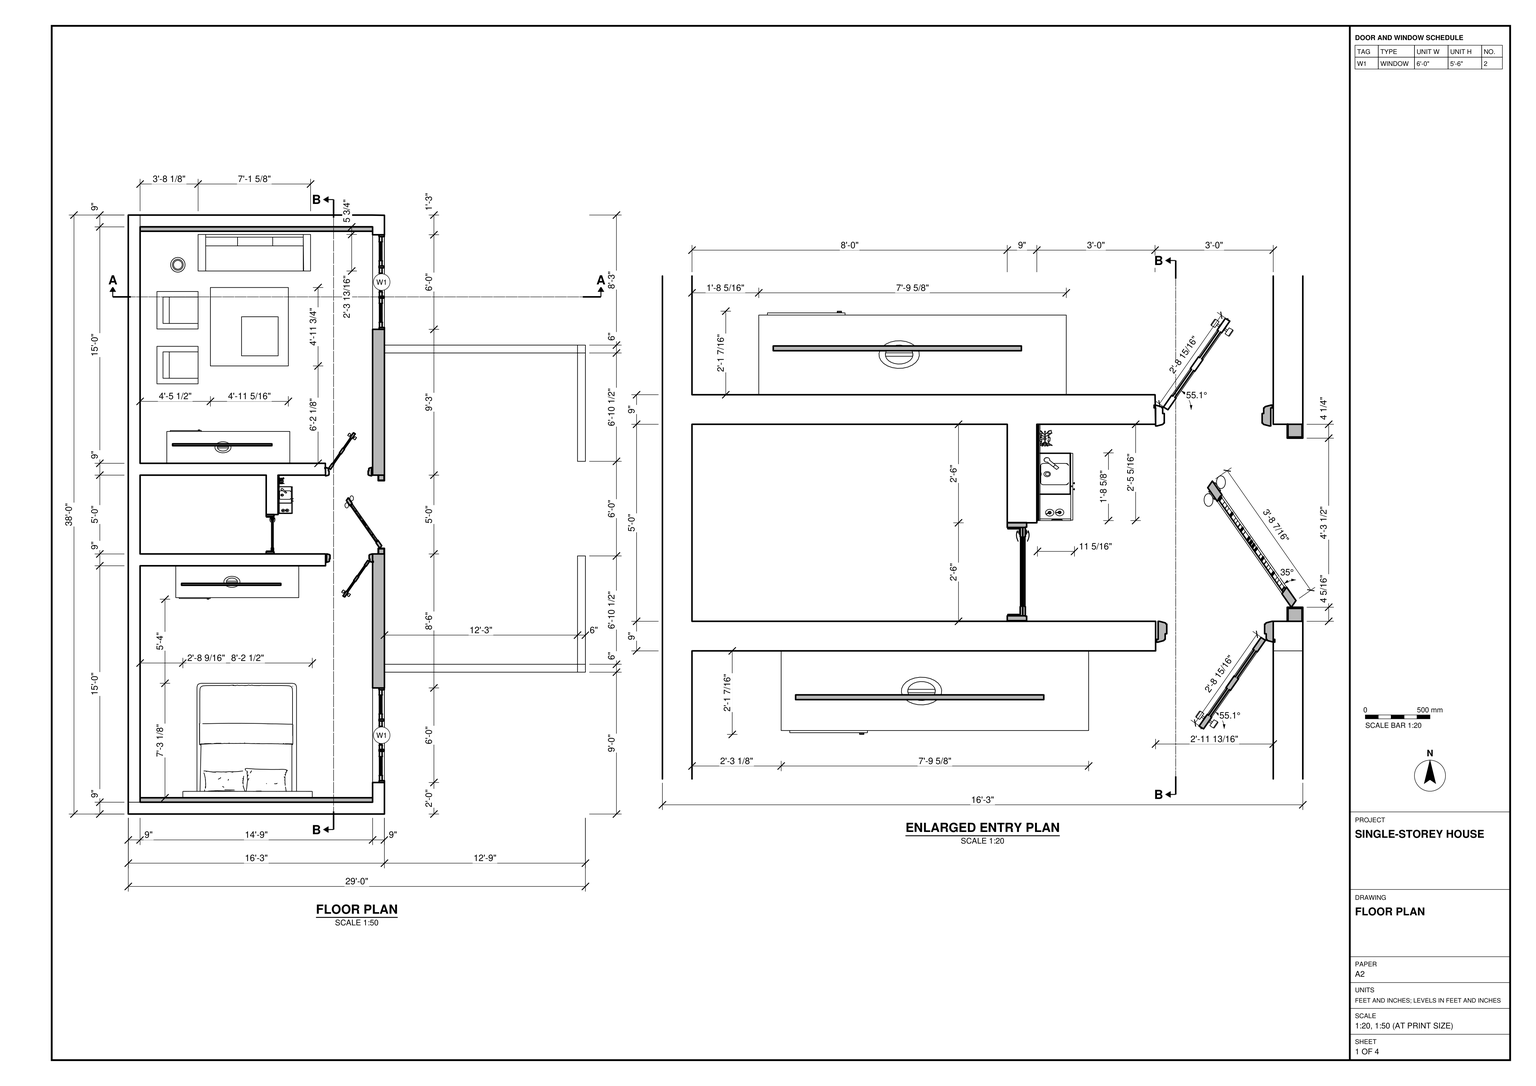
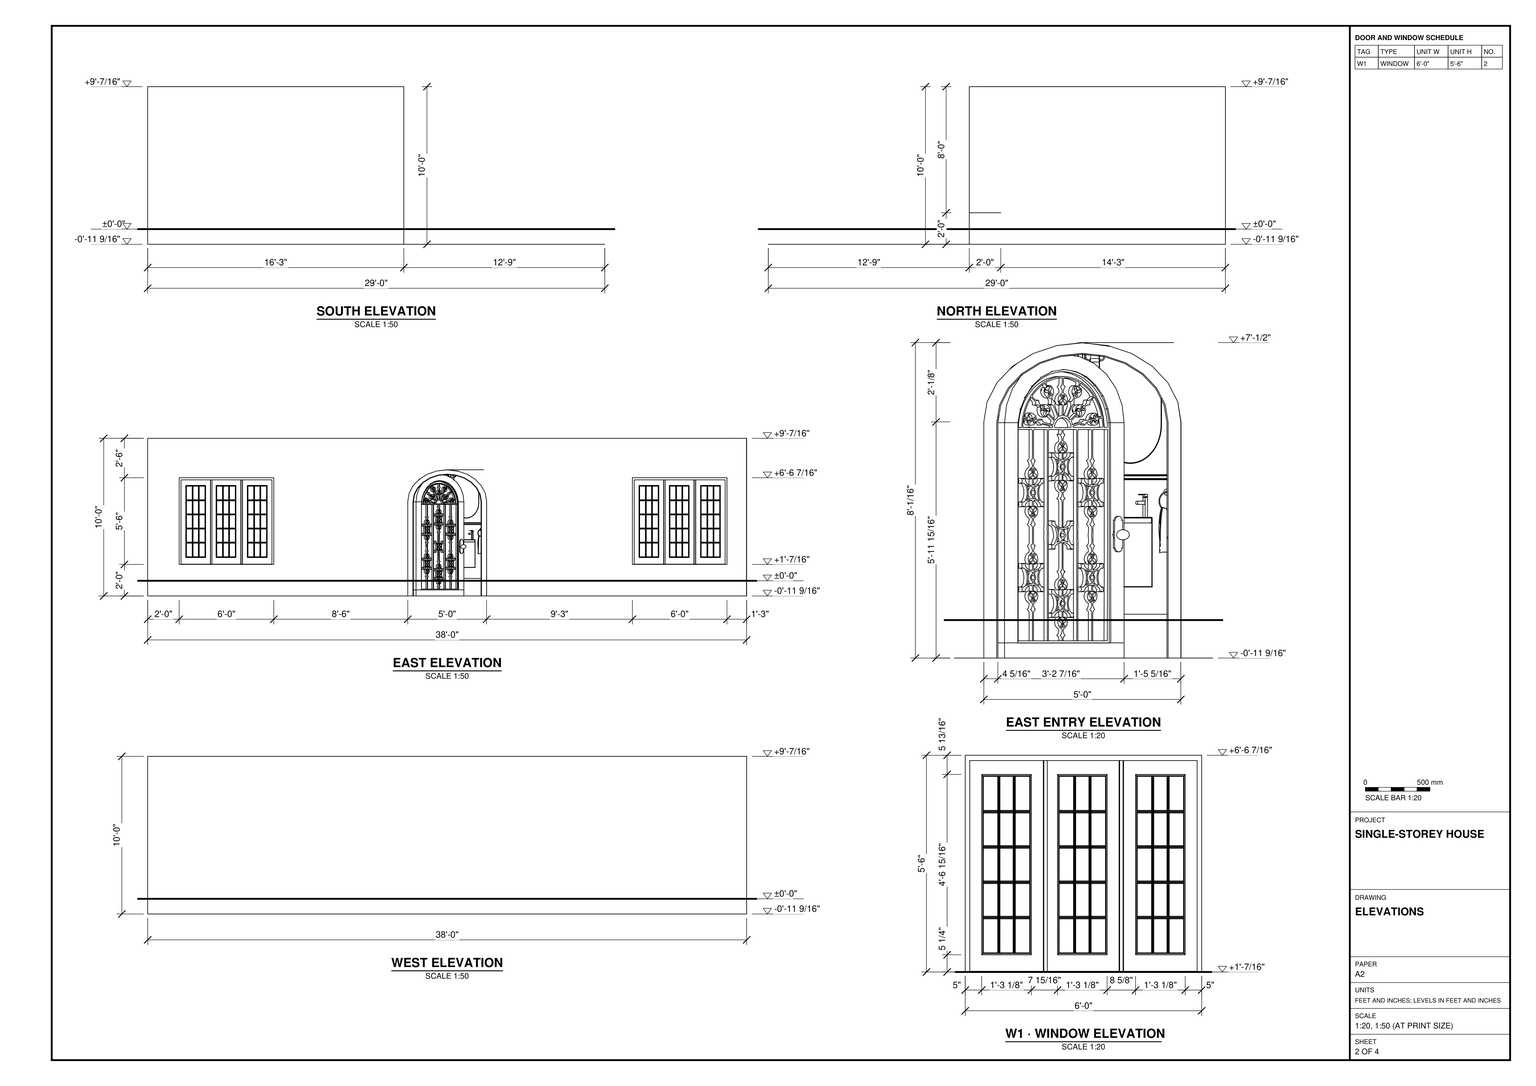
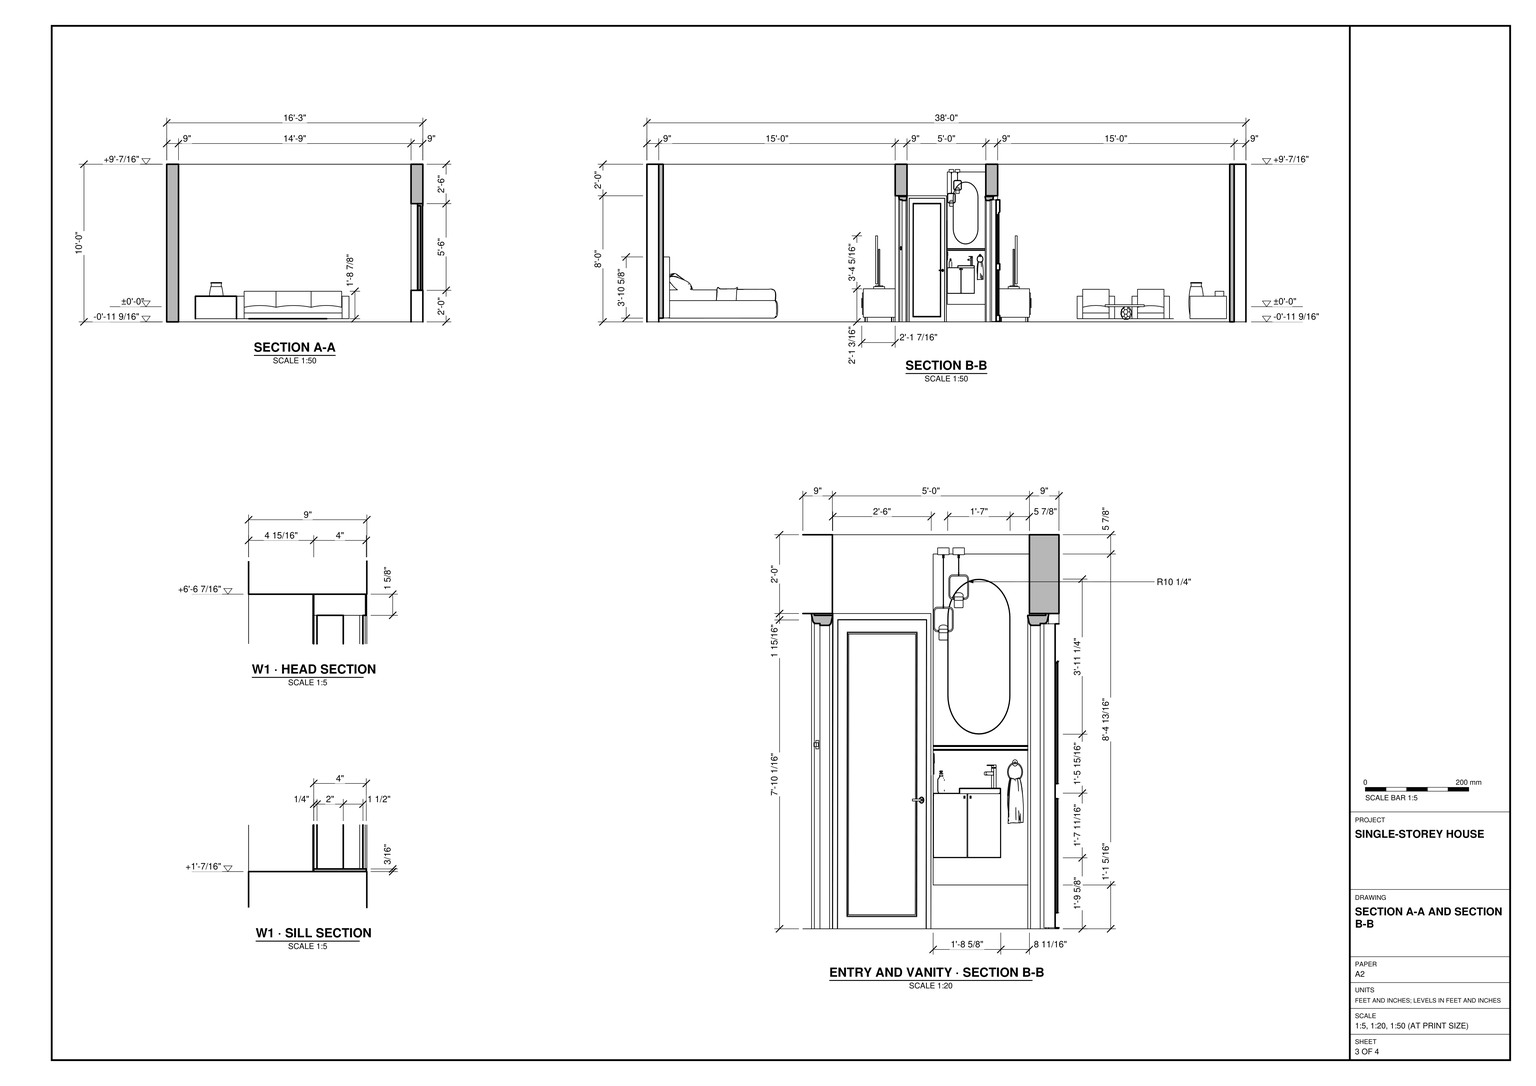
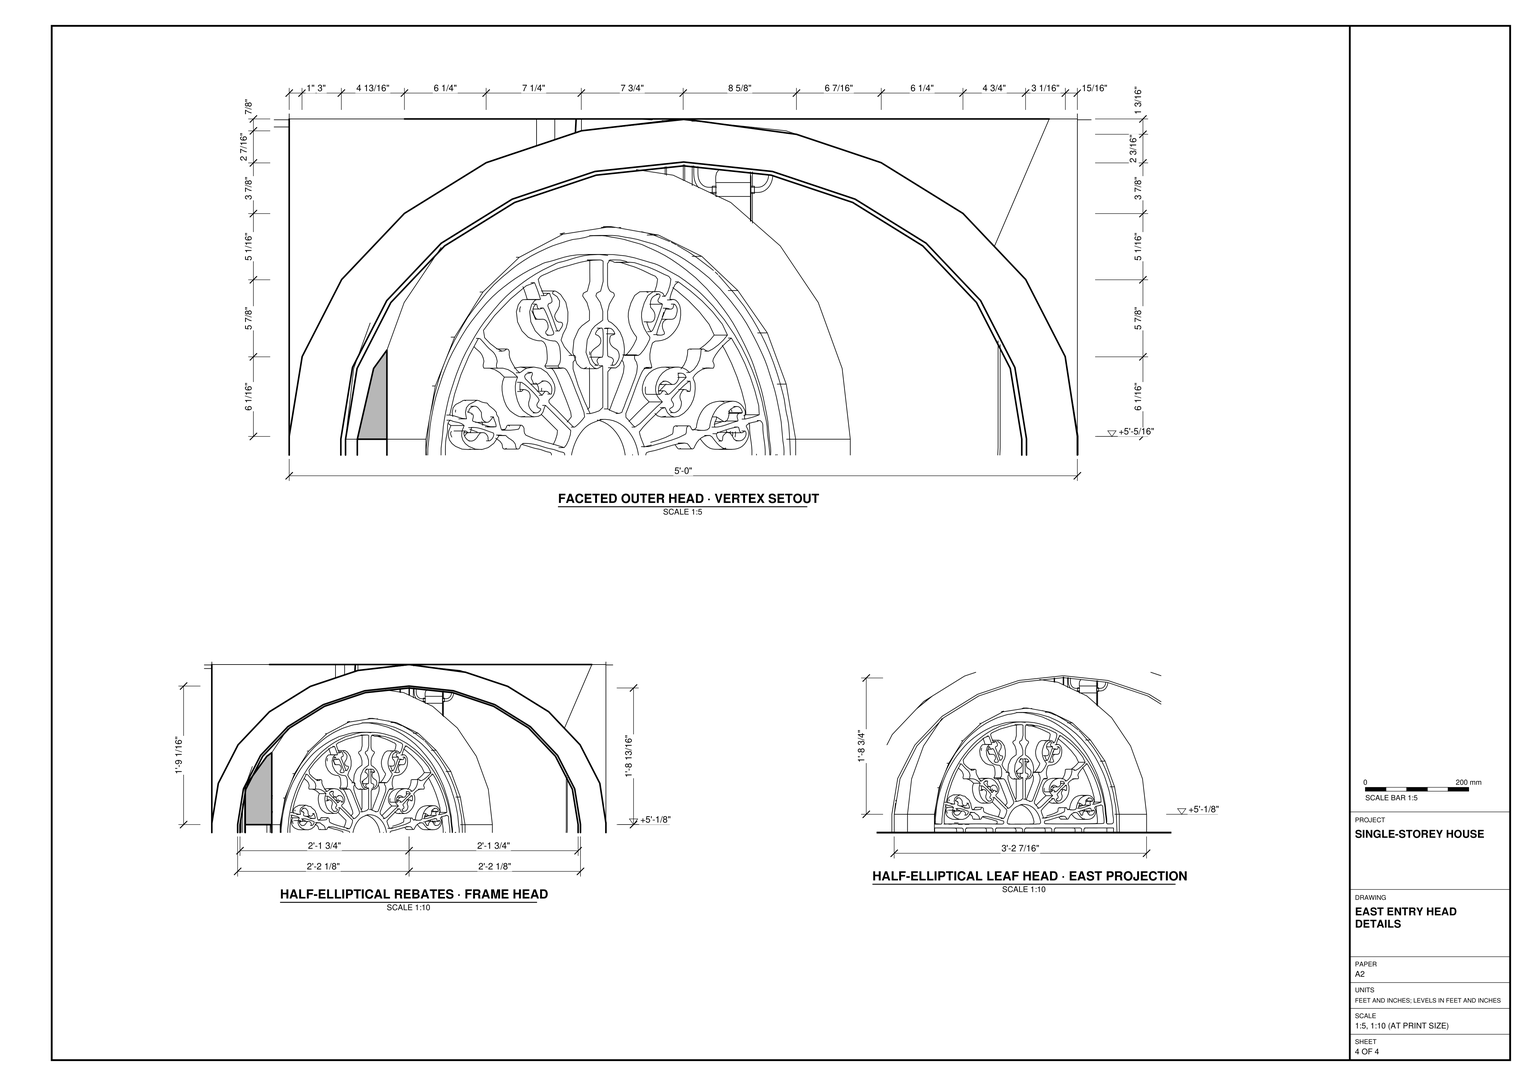
Build the house shown in task_files/diagram_01.pdf in SketchUp. Work in feet and inches. Use ±0'-0" as the ground-floor datum and follow the sections for the wall tops, window sills and floor position relative to that datum. The overall model is 29'-0" wide, 38'-0" long and 10'-0" high. The enclosed house is 16'-3" wide; the outline projecting from its east side accounts for the rest of the width. Follow the plan for its returns and the gap opposite the entrance.

Model the floor and the walls at their drawn thicknesses. Place the living room at the north end and the bedroom at the south end, with the entry and washbasin area between them. Use the enlarged entry plan for the partition returns, door positions and swing directions. Form the arched entrance and place a framed, divided-light window on either side of it, following the east elevation.

Set the sofa against the north wall and arrange the chairs and low table as drawn. Place the bed with its head against the south wall. Fit a television console against each room's entry-side partition, and include the vanity, basin and mirror in the entry recess. Decor and loose items may be any suitable library components. Keep shell elements and individual furniture or joinery pieces in separate groups or components, and use components for repeated parts. Save one SketchUp model as output_files/furnished_single_storey_house_with_arched_entry.skp.

# SketchUp Ruby script. Lengths in inches.
U = 1.inch
M = Sketchup.active_model
def pt(a) = Geom::Point3d.new(a.map { |v| v * U })
def face(e, loops, mat)
  f = e.add_face(loops[0].map { |a| pt(a) })
  loops[1..].each { |l| e.add_face(l.map { |a| pt(a) }).erase! }
  f.material = f.back_material = mat if mat
  f
end
# faces: each face lists its corners as indices into pts; further lists are holes
def faces(e, pts, list, mat = nil) = list.each { |f| face(e, (f[0].is_a?(Array) ? f : [f]).map { |l| l.map { |i| pts[i] } }, mat) }
# xy, xz, yz: faces in a plane at the given z, y or x. An outline is a flat list of corners, or four numbers for a rectangle; further outlines are holes
def ring(l) = l.size == 4 ? [[l[0], l[1]], [l[2], l[1]], [l[2], l[3]], [l[0], l[3]]] : l.each_slice(2).to_a
def flat(e, list, mat, &to3) = list.each { |f| face(e, (f[0].is_a?(Array) ? f : [f]).map { |l| ring(l).map { |u, v| to3.(u, v) } }, mat) }
def xy(e, z, list, mat = nil) = flat(e, list, mat) { |x, y| [x, y, z] }
def xz(e, y, list, mat = nil) = flat(e, list, mat) { |x, z| [x, y, z] }
def yz(e, x, list, mat = nil) = flat(e, list, mat) { |y, z| [x, y, z] }
def lines(e, pts, list) = list.each { |a, b| e.add_line(pt(pts[a]), pt(pts[b])) }
# prism: a flat outline (further loops are holes) pulled along v
def prism(e, loops, v, mat = nil)
  f = face(e, loops, mat); d = Geom::Vector3d.new(v.map { |x| x * U })
  f.pushpull(f.normal.samedirection?(d) ? d.length : -d.length)
end
def box(e, o, s, mat = nil) = prism(e, [[o, [o[0] + s[0], o[1], o[2]], [o[0] + s[0], o[1] + s[1], o[2]], [o[0], o[1] + s[1], o[2]]]], [0, 0, s[2]], mat)
def at(x, y, z, deg = 0) = Geom::Transformation.translation(pt([x, y, z])) * Geom::Transformation.rotation(ORIGIN, Z_AXIS, deg.degrees)
def axes(o, x, y, z) = Geom::Transformation.new([*x, 0, *y, 0, *z, 0, *pt(o).to_a, 1])
def part(name) = M.definitions.add(name)
# library, detail: a bought-in or finely detailed component or shape, given as its bounding box
def library(name, o, s) = part(name).tap { |d| box(d.entities, o, s) }
def detail(e, o, s) = box(e.add_group.entities, o, s)
def put(e, d, t, mat = nil) = e.add_instance(d, t).tap { |i| i.material = mat if mat }
def group(e, t, mat = nil) = e.add_group.tap { |g| g.transformation = t; g.material = mat if mat }.entities
root = M.entities
M.materials.add("[Beadboard]").color = [218, 143, 90]
M.materials.add("[Color M02]").color = [198, 198, 198]
M.materials.add("[Color M05]").color = [114, 114, 114]
M.materials.add("[Color M06]").color = [86, 86, 86]
M.materials.add("[Color_003]8").color = [199, 191, 184]
M.materials.add("[Color_A01]5").color = [191, 191, 191]
M.materials.add("[Color_A01]7").color = [193, 189, 163]
M.materials.add("[Color_A07]3").color = [188, 183, 174]
M.materials.add("[Ornate Tile 01]").color = [202, 202, 202]
c1 = library("BED 7",[-211.22,-92.85,196.6875],[87.15,98.53,46.62])
c2 = library("rack com tv",[110.42,162.32,-6.69],[191.73,75.99,125.98])
c3 = library("sofa set1",[-89.36,-29.2,-0.92],[221.25,236.08,46.83])
c4 = library("Раковина зеркало",[0,0,0],[11.3,36.42,102.67])
c5 = library("Three-panel window",[0.125,0,0],[4,104,82])
c6 = library("Group\#22",[0,0,0],[5.99,4.27,3.3])
c7 = library("Group\#8",[0,0,0],[6.69,30,96])
c8 = library("Group\#6",[-3,-0.25,0],[42,4.75,83.03])
c9 = library("Group\#7",[0,-2.02,0],[36,8.06,80])
xy(root,0,[[195,108,342,114],[342,108,348,114],[342,114,348,196.5],[342,268.5,348,351],[195,351,342,357],
  [342,351,348,357],[186,443.61,186.12,447],[9,443.67,186,447],[9,447,186,447.0625]])
xy(root,0,[[0,9,0,456,9,456,9,267,150,267,150.17,258,114,258,114,228,105,228,105,258,9,258,9,198,150.17,198,150.17,189,9,189,9,9],[186,189,195,198]],"[Color M02]")
xy(root,0,[[150.47,191.65,150.875,191.65,152.53,192.09,152.58,192.11,152.625,192.13,152.67,192.16,152.71,192.19,152.75,192.23,152.78,192.27,152.8125,192.31,152.84,192.36,152.86,192.4,152.875,192.45,152.89,192.51,153.09,192.51,153.09,194.21,153.57,194.21,153.57,197.15,153.36,197.15,153.35,197.2,153.31,197.3,153.28,197.34,153.25,197.39,153.18,197.46,153.1,197.52,153.05,197.54,153,197.5625,151.34,198,150.94,198,150.94,192.51,150.47,192.51],[186.07,191.65,186.47,191.65,186.47,192.51,186,192.51,186,198,185.6,198,183.9375,197.5625,183.89,197.54,183.84,197.52,183.76,197.46,183.69,197.39,183.66,197.34,183.63,197.3,183.61,197.25,183.6,197.2,183.58,197.15,183.37,197.15,183.37,194.21,183.85,194.21,183.85,192.51,184.05,192.51,184.07,192.45,184.08,192.4,184.11,192.36,184.13,192.31,184.16,192.27,184.2,192.23,184.23,192.19,184.27,192.16,184.32,192.13,184.36,192.11,184.41,192.09]],"[Color M05]")
xy(root,2.82,[[9,9,186,12.39]])
xy(root,24,[[186,369,195,441]])
xy(root,24,[[186,24,195,96]],"[Color M02]")
xy(root,54.78,[[153.05,192.97,153.09,193.86]],"[Color M05]")
xy(root,55.49,[[153.05,192.37,153.09,192.51],[153.05,192.51,153.09,192.97],[152.64,193.1,153.05,193.74],[153.05,193.1,153.09,193.74]],"[Color M05]")
xy(root,56.65,[[153.05,192.37,153.09,192.51],[153.05,192.51,153.09,192.97],[152.64,193.1,153.05,193.74],[153.05,193.1,153.09,193.74]],"[Color M05]")
xy(root,57.36,[[153.05,192.97,153.09,193.86]],"[Color M05]")
xy(root,90,[[186,24,195,96],[186,369,195,441]],"[Color M02]")
xy(root,92.4,[[153.57,194.21,183.37,197.15]],"[Color M05]")
xy(root,92.96,[[153.09,192.51,183.85,194.21]],"[Color M05]")
xy(root,95.45,[[150.94,192.51,186,198]],"[Color M05]")
xy(root,96,[[150.17,189,186,198],[105,198,114,228],[150.17,258,150,267,186,267,186,258]])
xy(root,96,[[150.47,191.65,186.47,192.51]],"[Color M05]")
xy(root,96.0625,[[186,198,190,202.32],[186,202.32,190.0625,206.77],[186,206.77,186,258,190.375,258,190.375,255.86,190.5,255.86,190.5,228,190.3125,228,190.3125,219.84,190.25,219.84,190.25,216.83,190.0625,216.83,190.0625,206.77],[190.0625,206.77,195,207.76],[190.0625,207.76,195,210.38],
  [190.0625,210.38,195,215.44],[190.0625,215.44,195,216.83],[190.25,216.83,195,218.22],[190.25,218.22,195,218.41],[190.25,218.41,195,219.84],
  [190.3125,219.84,195,220.25],[190.3125,220.25,195,221.34],[190.3125,221.34,195,228],[190.5,228,194.75,255.86],[190.375,255.86,190.5,258],
  [190.5,255.86,190.8125,258]])
xy(root,120,[[9,9,186,12.39],[9,447,186,447.0625]])
xy(root,120,[[[0,0,186,0,186,9,9,9,9,189,186,189,186,114,195,114,195,258,186,258,186,198,114,198,114,258,195,258,195,351,186,351,186,267,9,267,9,447.0625,186,447.0625,186,357,195,357,195,455.85,186,456,0,456],[9,198,105,258]],[186,0,195,108],[186,108,195,114],[186,351,195,357]],"[Color M02]")
xy(root,120.01,[[9,443.67,186,447.0625]])
xz(root,0,[[0,0,186,120],[186,0,195,120]])
xz(root,9,[[9,0,186,2.82]])
xz(root,9,[[9,2.82,186,120]],"[Color_A01]7")
xz(root,12.39,[[9,2.82,186,120]],"[Color_A01]5")
xz(root,24,[[186,24,195,90]],"[Color M02]")
xz(root,96,[[186,24,195,90]],"[Color M02]")
xz(root,189,[[9,0,150.17,0,150.17,96,186,96,186,120,9,120]],"[Color M02]")
xz(root,191.65,[[150.47,0,150.47,96,186.47,96,186.47,0,186.07,0,186.07,95.53,150.875,95.53,150.875,0]],"[Color M05]")
xz(root,192.37,[[153.05,55.49,153.09,56.65]],"[Color M05]")
xz(root,192.51,[[150.47,0,150.94,0,150.94,95.45,186,95.45,186,0,186.47,0,186.47,96,150.47,96],[152.89,0,152.89,93.19,184.05,93.19,184.05,0,183.85,0,183.85,92.96,153.09,92.96,153.09,56.65,153.05,56.65,153.05,55.49,153.09,55.49,153.09,0]],"[Color M05]")
xz(root,192.97,[[153.05,54.78,153.09,55.49],[153.05,56.65,153.09,57.36]],"[Color M05]")
xz(root,193.1,[[152.64,55.49,153.05,56.65],[153.05,55.49,153.09,56.65]],"[Color M05]")
xz(root,193.74,[[152.64,55.49,153.05,56.65],[153.05,55.49,153.09,56.65]],"[Color M05]")
xz(root,193.86,[[153.05,54.78,153.09,57.36]],"[Color M05]")
xz(root,194.21,[[153.09,0,153.09,92.96,183.85,92.96,183.85,0,183.37,0,183.37,92.4,153.57,92.4,153.57,0]],"[Color M05]")
xz(root,197.15,[[153.36,0,153.57,0,153.57,92.4,183.37,92.4,183.37,0,183.58,0,183.58,92.65,153.36,92.65]],"[Color M05]")
xz(root,198,[[186,0,186,96.0625,190,96.0625,190,71.91,195,71.91,195,0],[190,71.91,194.125,96.0625]])
xz(root,198,[[105,0,105,96,114,96,114,120,186,120,186,96,150.17,96,150.17,0]],"[Color M02]")
xz(root,198,[[150.94,0,151.34,0,151.34,94.98,185.6,94.98,185.6,0,186,0,186,95.45,150.94,95.45]],"[Color M05]")
xz(root,198,[[9,0,105,120]],"[Ornate Tile 01]")
xz(root,216.83,[[190.0625,94.02,190.25,96.0625]])
xz(root,228,[[105,0,114,96]])
xz(root,258,[[186,0,195,0,195,71.91,190.375,71.91,190.375,96.0625,186,96.0625],[190.375,71.91,190.5,96.0625],[190.5,71.91,190.8125,96.0625]])
xz(root,258,[[114,0,150.17,0,150.17,96,186,96,186,120,114,120]],"[Color M02]")
xz(root,258,[[9,0,105,120]],"[Ornate Tile 01]")
xz(root,267,[[9,0,9,120,186,120,186,96,150,96,150,0]],"[Color M02]")
xz(root,369,[[186,24,195,90]],"[Color M02]")
xz(root,441,[[186,24,195,90]],"[Color M02]")
xz(root,443.67,[[9,0,186,120.01]],"[Color_003]8")
xz(root,447,[[9,0,186,120]],"[Color_A07]3")
xz(root,447.0625,[[9,0,186,120],[9,120,186,120.01]],"[Color_A07]3")
xz(root,456,[[0,0,9,120],[9,0,186,120]],"[Color M02]")
yz(root,0,[[0,0,456,120]],"[Color M02]")
yz(root,9,[[267,0,443.67,120],[443.67,0,447,120],[447,0,447.0625,120],[9,2.82,12.39,120],[443.67,120,447.0625,120.01]])
yz(root,9,[[9,0,189,0,189,120,12.39,120,12.39,2.82,9,2.82]],"[Color M02]")
yz(root,9,[[198,0,258,120]],"[Ornate Tile 01]")
yz(root,105,[[228,0,228,96,198,96,198,120,258,120,258,0]],"[Ornate Tile 01]")
yz(root,114,[[228,0,258,0,258,120,198,120,198,96,228,96]],"[Beadboard]")
yz(root,150.17,[[189,0,198,96]])
yz(root,150.47,[[191.65,0,192.51,96]],"[Color M05]")
yz(root,150.94,[[192.51,0,198,95.45]],"[Color M05]")
yz(root,152.64,[[193.1,55.49,193.74,56.65]],"[Color M05]")
yz(root,153.05,[[[192.97,54.78,192.97,55.49,192.51,55.49,192.51,56.65,192.97,56.65,192.97,57.36,193.86,57.36,193.86,54.78],[193.1,55.49,193.74,56.65]],[192.37,55.49,192.51,56.65]],"[Color M05]")
yz(root,153.09,[[192.51,0,192.51,55.49,192.97,55.49,192.97,54.78,193.86,54.78,193.86,57.36,192.97,57.36,192.97,56.65,192.51,56.65,192.51,92.96,194.21,92.96,194.21,0],[[192.97,54.78,193.86,54.78,193.86,57.36,192.97,57.36,192.97,56.65,192.37,56.65,192.37,55.49,192.97,55.49],[193.1,55.49,193.74,56.65]]],"[Color M05]")
yz(root,153.57,[[194.21,0,197.15,92.4]],"[Color M05]")
yz(root,183.37,[[194.21,0,197.15,92.4]],"[Color M05]")
yz(root,183.85,[[192.51,0,194.21,92.96]],"[Color M05]")
yz(root,186,[[189,0,192.51,0,192.51,95.45,198,95.45,198,96,189,96],[258,0,267,96],[267,0,351,120],[351,0,357,120],[[357,0,443.67,120],[369,24,441,90]],
  [443.67,0,447,120],[447,0,447.0625,120],[9,2.82,12.39,120],[443.67,120,447.0625,120.01]])
yz(root,186,[[[9,0,9,2.82,12.39,2.82,12.39,120,108,120,108,0],[24,24,96,90]],[108,0,114,120],[114,0,189,120],[198,96.0625,258,120]],"[Color M02]")
yz(root,186,[[192.51,0,198,95.45]],"[Color M05]")
yz(root,186.47,[[191.65,0,192.51,96]],"[Color M05]")
yz(root,190,[[198,71.91,198,96.0625,202.32,96.0625,203.16,85.07,201.99,83.84,198.99,77.97]],"[Color M02]")
yz(root,190.0625,[[203.16,85.07,204.0625,86.02,205.71,87.75,206.77,88.87,208.08,89.68,210.38,91.11,213,92.73,214.22,93.14,216.83,94.02,216.83,96.0625,202.32,96.0625]],"[Color M02]")
yz(root,190.25,[[216.83,94.02,217.5,94.24,218.22,94.48,218.22,96.0625,216.83,96.0625],[218.22,94.48,218.22,96.0625,219.84,96.0625,219.79,95.01,218.41,94.55]])
yz(root,190.3125,[[219.79,95.01,220.25,95.16,220.25,96.0625,219.84,96.0625],[220.25,95.16,221.34,95.29,228,96.0625,220.25,96.0625]])
yz(root,190.5,[[258,71.91,257.07,77.97,254.07,83.84,251.68,86.35,249.29,88.87,243.0625,92.73,236.61,94.89,228,96.0625,258,96.0625]],"[Color M02]")
yz(root,190.8125,[[258,71.91,257.07,77.97,254.07,83.84,251.68,86.35,255.86,96.0625,258,96.0625]])
yz(root,194.125,[[198,71.91,198,96.0625,203.16,85.07,201.99,83.84,198.99,77.97]])
yz(root,194.75,[[249.29,88.87,255.86,96.0625,243.0625,92.73],[243.0625,92.73,255.86,96.0625,228,96.0625,236.61,94.89]])
yz(root,195,[[205.71,87.75,205.88,87.89,206.18,88.14,206.93,88.77,206.77,88.87,205.98,88.03],[205.88,87.89,206.05,88.03,206.18,88.14],[206.05,88.03,208.08,89.68,207.9375,89.59,206.18,88.14],[206.18,88.14,207.9375,89.59,207.8,89.51,206.93,88.77],[206.93,88.77,207.11,89.08,206.77,88.87],
  [206.93,88.77,207.8,89.51,207.11,89.08]])
yz(root,195,[[[0,0,198,120],[24,24,96,90]],[[258,0,455.85,0,455.85,120,198,120,198,96.0625,255.86,96.0625,251.68,86.35,254.07,83.84,257.07,77.97,258,71.91],[369,24,441,90]],[198,71.91,198.99,77.97,201.99,83.84,203.16,85.07,198,96.0625],[203.16,85.07,198,96.0625,202.32,96.0625],[203.16,85.07,205.71,87.75,205.98,88.03,206.77,88.87,207.11,89.08,207.8,89.51,207.9375,89.59,208.08,89.68,210.38,91.11,213,92.73,215.44,93.55,215.44,96.0625,202.32,96.0625],
  [251.68,86.35,255.86,96.0625,249.29,88.87],[249.29,88.87,255.86,96.0625,228,96.0625,229,95.93,236.61,94.89,243.0625,92.73],[215.44,93.55,216.83,94.02,218.22,94.48,218.22,96.0625,215.44,96.0625],[218.22,94.48,218.41,94.55,219.79,95.01,219.84,96.0625,218.22,96.0625],[219.79,95.01,220.25,95.16,221.34,95.29,228,96.0625,219.84,96.0625]],"[Color M02]")
p = [[150.875,191.65,95.53],[152.53,192.09,93.6],[152.53,192.09,0],[150.875,191.65,0],[186.07,191.65,0],[184.41,192.09,0],
  [184.41,192.09,93.6],[186.07,191.65,95.53],[152.58,192.11,93.55],[152.58,192.11,0],[152.625,192.13,93.5],[152.67,192.16,93.45],
  [152.67,192.16,0],[152.625,192.13,0],[184.32,192.13,0],[184.27,192.16,0],[184.27,192.16,93.45],[184.32,192.13,93.5],
  [184.36,192.11,0],[184.36,192.11,93.55],[152.71,192.19,93.4],[152.71,192.19,0],[152.75,192.23,93.36],[152.75,192.23,0],
  [152.78,192.27,93.32],[152.78,192.27,0],[184.2,192.23,0],[184.16,192.27,0],[184.16,192.27,93.32],[184.2,192.23,93.36],
  [184.23,192.19,0],[184.23,192.19,93.4],[152.8125,192.31,93.28],[152.84,192.36,93.25],[152.84,192.36,0],[152.8125,192.31,0],
  [184.13,192.31,0],[184.13,192.31,93.28],[184.11,192.36,0],[184.11,192.36,93.25],[152.86,192.4,93.23],[152.86,192.4,0],
  [152.875,192.45,93.21],[152.875,192.45,0],[184.08,192.4,0],[184.08,192.4,93.23],[184.07,192.45,0],[184.07,192.45,93.21],
  [152.89,192.51,93.19],[152.89,192.51,0],[184.05,192.51,0],[184.05,192.51,93.19],[153.36,197.15,92.65],[153.35,197.2,92.66],
  [153.35,197.2,0],[153.36,197.15,0],[183.58,197.15,0],[183.6,197.2,0],[183.6,197.2,92.66],[183.58,197.15,92.65],
  [153.33,197.25,92.68],[153.33,197.25,0],[153.31,197.3,92.7],[153.31,197.3,0],[183.61,197.25,0],[183.63,197.3,0],
  [183.63,197.3,92.7],[183.61,197.25,92.68],[153.28,197.34,92.73],[153.25,197.39,92.77],[153.25,197.39,0],[153.28,197.34,0],
  [183.66,197.34,0],[183.66,197.34,92.73],[183.69,197.39,0],[183.69,197.39,92.77],[153.22,197.42,92.81],[153.18,197.46,92.85],
  [153.18,197.46,0],[153.22,197.42,0],[183.72,197.42,0],[183.76,197.46,0],[183.76,197.46,92.85],[183.72,197.42,92.81],
  [153.05,197.54,93],[153,197.5625,93.06],[153,197.5625,0],[153.05,197.54,0],[153.14,197.49,92.9],[153.1,197.52,92.95],
  [153.1,197.52,0],[153.14,197.49,0],[183.8,197.49,0],[183.84,197.52,0],[183.84,197.52,92.95],[183.8,197.49,92.9],
  [183.89,197.54,0],[183.89,197.54,93],[183.9375,197.5625,0],[183.9375,197.5625,93.06],[151.34,198,94.98],[151.34,198,0],
  [185.6,198,0],[185.6,198,94.98],[150,267,0],[150,267,96],[150.17,258,96],[150.17,258,0],
  [195,455.85,0],[186,456,0],[186,456,120],[195,455.85,120],[195,455.85,24],[190,198.99,77.97],
  [190,198,71.91],[194.125,198,71.91],[194.125,198.99,77.97],[195,198,71.91],[195,198.99,77.97],[190.5,258,71.91],
  [190.5,257.07,77.97],[190.375,257.07,77.97],[190.375,258,71.91],[190.8125,257.07,77.97],[190.8125,258,71.91],[195,257.07,77.97],
  [195,258,71.91],[190,201.99,83.84],[194.125,201.99,83.84],[195,201.99,83.84],[190.5,254.07,83.84],[190.375,254.07,83.84],
  [190.8125,254.07,83.84],[195,254.07,83.84],[190,203.16,85.07],[194.125,203.16,85.07],[190.0625,203.16,85.07],[195,203.16,85.07],
  [190.5,251.68,86.35],[190.375,251.68,86.35],[190.8125,251.68,86.35],[195,251.68,86.35],[190,202.32,96.0625],[190.0625,202.32,96.0625],
  [195,205.71,87.75],[190.18,205.71,87.75],[190.0625,204.0625,86.02],[190.0625,205.71,87.75],[190.5,249.29,88.87],[194.75,249.29,88.87],
  [195,249.29,88.87],[190.25,206.77,88.87],[190.0625,206.77,88.87],[195,206.77,88.87],[195,205.98,88.03],[190.25,208.08,89.68],
  [190.0625,208.08,89.68],[195,208.08,89.68],[195,207.11,89.08],[195,207.8,89.51],[195,207.9375,89.59],[190.5,243.0625,92.73],
  [194.75,243.0625,92.73],[195,243.0625,92.73],[190.25,210.38,91.11],[190.0625,210.38,91.11],[195,210.38,91.11],[190.25,213,92.73],
  [190.0625,213,92.73],[195,213,92.73],[190.25,214.22,93.14],[190.0625,214.22,93.14],[195,214.22,93.14],[190.5,236.61,94.89],
  [194.75,236.61,94.89],[195,236.61,94.89],[190.25,216.83,94.02],[190.0625,216.83,94.02],[195,216.83,94.02],[195,215.44,93.55],
  [195,218.22,94.48],[190.25,218.22,94.48],[190.25,217.5,94.24],[195,218.41,94.55],[190.25,218.41,94.55],[195,219.79,95.01],
  [190.25,219.79,95.01],[190.3125,219.79,95.01],[190.5,228,96.0625],[194.75,228,96.0625],[195,229,95.93],[195,228,96.0625],
  [190.25,219.84,96.0625],[190.3125,219.84,96.0625],[195,220.25,95.16],[190.3125,220.25,95.16],[195,219.84,96.0625],[195,221.34,95.29],
  [190.3125,221.34,95.29],[190.3125,228,96.0625],[171,455.85,24],[186,483.8,0],[186.12,483.8,0],[186,574.61,0],
  [186.12,574.61,0],[190.25,220.25,95.16],[190.25,223.6,95.52],[190.25,227.08,95.89],[186,224.53,96.0625],[195,228.63,95.93]]
faces(root,p,[[0,1,2,3],[4,5,6,7],[1,8,9,2],[10,11,12,13],[8,10,13,9],[14,15,16,17],[18,14,17,19],[5,18,19,6],
  [11,20,21,12],[20,22,23,21],[22,24,25,23],[26,27,28,29],[30,26,29,31],[15,30,31,16],[32,33,34,35],[24,32,35,25],
  [27,36,37,28],[36,38,39,37],[33,40,41,34],[40,42,43,41],[38,44,45,39],[44,46,47,45],[42,48,49,43],[46,50,51,47],
  [52,53,54,55],[56,57,58,59],[53,60,61,54],[60,62,63,61],[64,65,66,67],[57,64,67,58],[68,69,70,71],[62,68,71,63],
  [65,72,73,66],[72,74,75,73],[76,77,78,79],[69,76,79,70],[80,81,82,83],[74,80,83,75],[84,85,86,87],[88,89,90,91],
  [89,84,87,90],[77,88,91,78],[92,93,94,95],[81,92,95,82],[93,96,97,94],[96,98,99,97],[85,100,101,86],[98,102,103,99],
  [59,58,53,52],[58,67,60,53],[67,66,62,60],[73,75,69,68],[66,73,68,62],[75,83,76,69],[83,82,77,76],[82,95,88,77],
  [94,97,84,89],[95,94,89,88],[97,99,85,84],[99,103,100,85],[39,45,40,33],[45,47,42,40],[47,51,48,42],[29,28,24,22],
  [28,37,32,24],[37,39,33,32],[17,16,11,10],[31,29,22,20],[16,31,20,11],[6,19,8,1],[19,17,10,8],[7,6,1,0]],"[Color M05]")
faces(root,p,[[104,105,106,107],[113,114,115,116],[117,118,116,115],[119,120,121,122],[119,120,123,124],[124,123,125,126],[127,113,116,128],[118,129,128,116],
  [120,130,131,121],[120,130,132,123],[123,132,133,125],[134,127,128,135,136],[129,137,135,128],[130,138,139,131],[130,138,140,132],[132,140,141,133],
  [134,142,143,136],[144,145,146,136,135,137],[147,146,145],[138,148,149,150,141,140],[147,145,151,152],[153,151,145,144,154],[152,151,155,156],[157,155,151,153,158,159,160],
  [148,161,162,149],[163,150,162],[150,149,162],[156,155,164,165],[166,164,155,157],[165,164,167,168],[169,167,164,166],[168,167,170,171],
  [172,170,167,169],[161,173,174,162],[163,162,175],[174,175,162],[171,170,176,177],[178,176,170,172,179],[178,180,181,182,176],[183,180,181,184],
  [185,183,184,186,187],[173,188,189,174],[190,175,174,189,191],[192,193,187,186],[185,194,195,187],[196,185,187,193],[194,197,198,195],[197,191,189,188,199,198]])
faces(root,p,[[108,109,110,111,112]],"[Color M02]")
lines(root,p,[[112,200],[201,202],[203,204],[134,146],[205,206],[206,207],[207,208],[186,205],[209,190]])
detail(root,[163.42,165.24,0.3],[20.19,27.83,92.57])
detail(root,[183.61,192.08,45.17],[0.4,0.43,0.91])
detail(root,[183.61,192.08,47.98],[0.4,0.43,0.67])
detail(root,[183.61,192.08,13.36],[0.4,0.43,0.68])
detail(root,[183.61,192.08,82.81],[0.4,0.43,0.7])
detail(root,[183.61,192.08,46.11],[0.4,0.43,0.91])
detail(root,[183.61,192.08,10.55],[0.4,0.43,0.91])
detail(root,[183.61,192.08,86.34],[0.4,0.43,0.68])
detail(root,[183.61,192.08,12.42],[0.4,0.43,0.91])
detail(root,[183.61,192.08,84.47],[0.4,0.43,0.91])
detail(root,[183.61,192.08,9.82],[0.4,0.43,0.71])
detail(root,[183.61,192.08,83.53],[0.4,0.43,0.91])
detail(root,[183.61,192.08,11.49],[0.4,0.43,0.91])
detail(root,[183.61,192.08,47.04],[0.4,0.43,0.91])
detail(root,[183.61,192.08,44.44],[0.4,0.43,0.71])
detail(root,[183.61,192.08,85.4],[0.4,0.43,0.92])
detail(root,[152.17,262.99,46.11],[0.4,0.42,0.91])
detail(root,[149.71,257.49,0],[36,6.35,96])
detail(root,[152.17,262.99,9.82],[0.4,0.42,0.71])
detail(root,[152.17,262.99,12.42],[0.4,0.42,0.91])
detail(root,[152.57,262.42,0.3],[20.19,27.83,92.57])
detail(root,[152.17,262.99,47.04],[0.4,0.42,0.91])
detail(root,[152.17,262.99,10.55],[0.4,0.42,0.91])
detail(root,[152.17,262.99,47.98],[0.4,0.42,0.67])
detail(root,[152.17,262.99,82.81],[0.4,0.42,0.7])
detail(root,[152.17,262.99,44.44],[0.4,0.42,0.71])
detail(root,[152.17,262.99,85.4],[0.4,0.42,0.92])
detail(root,[152.17,262.99,13.36],[0.4,0.42,0.68])
detail(root,[152.17,262.99,86.34],[0.4,0.42,0.68])
detail(root,[152.17,262.99,83.53],[0.4,0.42,0.91])
detail(root,[152.17,262.99,84.47],[0.4,0.42,0.91])
detail(root,[152.17,262.99,45.17],[0.4,0.42,0.91])
detail(root,[152.17,262.99,11.49],[0.4,0.42,0.91])
put(root,c1,at(47.22,223.61,-193.87,90))
put(root,c2,axes([-17.77,109.19,3.48],[0.48836,0,0],[0,0.33489,0],[0,0,0.52]))
put(root,c2,axes([-24.59,346.81,3.48],[0.48836,0,0],[0,-0.33489,0],[0,0,0.52]))
put(root,c3,axes([91.54,427.16,2.41],[-0.52853,0,0],[0,-0.48162,0],[0,0,0.6006]))
put(root,c4,axes([114.1875,228.68,13.33],[1,0,0],[0,0.8051,0],[0,0,1]))
put(root,c5,axes([195,96,24],[-1,-0.00174,0],[0.0012,-0.69231,0],[0,0,0.80488]),"[Color M05]")
put(root,c5,axes([195,441,24],[-1,-0.00174,0],[0.0012,-0.69231,0],[0,0,0.80488]),"[Color M05]")
put(root,c6,axes([166.46,163.48,40.05],[-0.91736,0.64144,0],[0.67387,0.87322,0],[0,0,1.16114]),"[Color M05]")
put(root,c6,axes([169.72,292.01,40.05],[0.91736,-0.64144,0],[-0.67387,-0.87322,0],[0,0,1.16114]),"[Color M05]")
put(root,c7,at(105,198.11,0))
put(root,c8,axes([194.75,202.29,0],[0,1.43,0],[-1,0,0],[0,0,1.15615]),"[Color M06]")
put(root,c9,axes([193.63,205.33,0],[-0.70711,1.01116,0],[-0.70711,-1.01116,0],[0,0,1.15615]),"[Color M05]")
